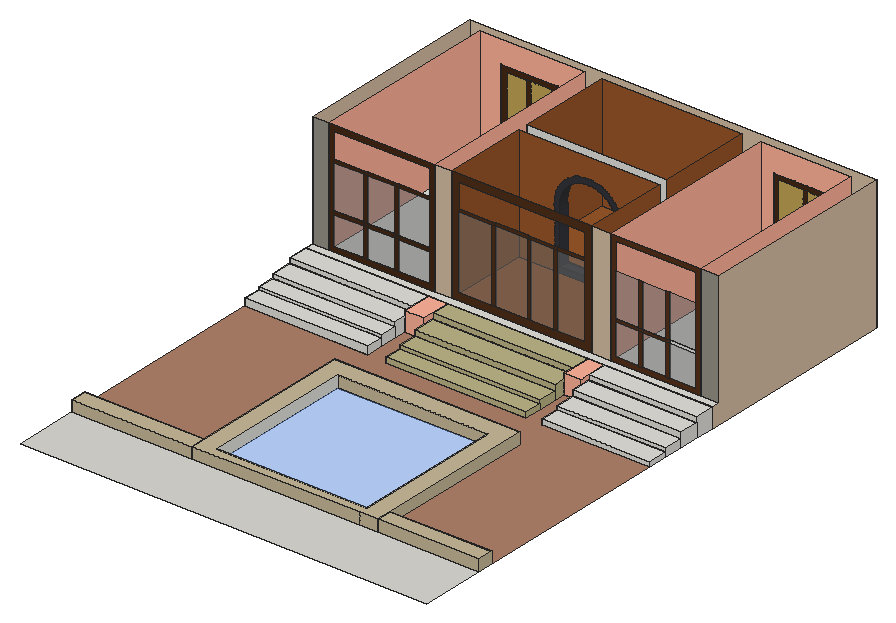
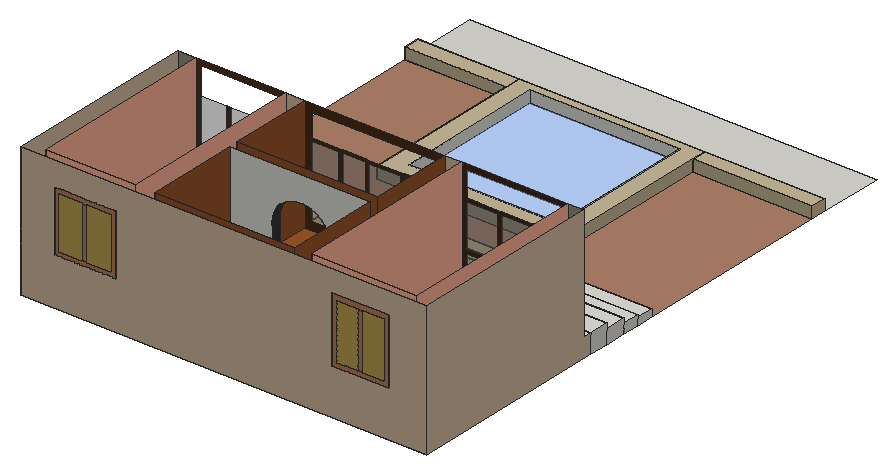
# SketchUp Ruby script. Lengths in inches.
U = 1.inch
M = Sketchup.active_model
def pt(a) = Geom::Point3d.new(a.map { |v| v * U })
def face(e, loops, mat)
  f = e.add_face(loops[0].map { |a| pt(a) })
  loops[1..].each { |l| e.add_face(l.map { |a| pt(a) }).erase! }
  f.material = f.back_material = mat if mat
  f
end
# faces: each face lists its corners as indices into pts; further lists are holes
def faces(e, pts, list, mat = nil) = list.each { |f| face(e, (f[0].is_a?(Array) ? f : [f]).map { |l| l.map { |i| pts[i] } }, mat) }
# xy, xz, yz: faces in a plane at the given z, y or x. An outline is a flat list of corners, or four numbers for a rectangle; further outlines are holes
def ring(l) = l.size == 4 ? [[l[0], l[1]], [l[2], l[1]], [l[2], l[3]], [l[0], l[3]]] : l.each_slice(2).to_a
def flat(e, list, mat, &to3) = list.each { |f| face(e, (f[0].is_a?(Array) ? f : [f]).map { |l| ring(l).map { |u, v| to3.(u, v) } }, mat) }
def xy(e, z, list, mat = nil) = flat(e, list, mat) { |x, y| [x, y, z] }
def xz(e, y, list, mat = nil) = flat(e, list, mat) { |x, z| [x, y, z] }
def yz(e, x, list, mat = nil) = flat(e, list, mat) { |y, z| [x, y, z] }
def lines(e, pts, list) = list.each { |a, b| e.add_line(pt(pts[a]), pt(pts[b])) }
# prism: a flat outline (further loops are holes) pulled along v
def prism(e, loops, v, mat = nil)
  f = face(e, loops, mat); d = Geom::Vector3d.new(v.map { |x| x * U })
  f.pushpull(f.normal.samedirection?(d) ? d.length : -d.length)
end
def box(e, o, s, mat = nil) = prism(e, [[o, [o[0] + s[0], o[1], o[2]], [o[0] + s[0], o[1] + s[1], o[2]], [o[0], o[1] + s[1], o[2]]]], [0, 0, s[2]], mat)
def at(x, y, z, deg = 0) = Geom::Transformation.translation(pt([x, y, z])) * Geom::Transformation.rotation(ORIGIN, Z_AXIS, deg.degrees)
def axes(o, x, y, z) = Geom::Transformation.new([*x, 0, *y, 0, *z, 0, *pt(o).to_a, 1])
def part(name) = M.definitions.add(name)
# library, detail: a bought-in or finely detailed component or shape, given as its bounding box
def library(name, o, s) = part(name).tap { |d| box(d.entities, o, s) }
def detail(e, o, s) = box(e.add_group.entities, o, s)
def put(e, d, t, mat = nil) = e.add_instance(d, t).tap { |i| i.material = mat if mat }
def group(e, t, mat = nil) = e.add_group.tap { |g| g.transformation = t; g.material = mat if mat }.entities
root = M.entities
M.materials.add("[Blinds Cloth Horizontal]").color = [192, 163, 85]
M.materials.add("[Color B02]").color = [255, 178, 153]
M.materials.add("[Formica Beige]").color = [211, 187, 149]
M.materials.add("[Formica Graystone]").color = [149, 146, 135]
M.materials.add("[Formica Laminate Dark]").color = [50, 53, 60]
M.materials.add("[Formica Laminate Light]").color = [213, 189, 164]
M.materials.add("[Marble Carrara Gold Floor Tile]").color = [225, 223, 217]
M.materials.add("[Pavers Driveway Brick]").color = [176, 130, 106]
M.materials.add("[Quartz Light Brown]").color = [199, 184, 152]
M.materials.add("[Terrazzo Tile Light]").color = [219, 217, 210]
M.materials.add("[Tile Ceramic Natural]").color = [189, 180, 134]
M.materials.add("[Translucent Glass Blue]").color = [100, 149, 237]
M.materials["[Translucent Glass Blue]"].alpha = 0.5
M.materials.add("[Translucent Glass Gray]").color = [128, 128, 128]
M.materials["[Translucent Glass Gray]"].alpha = 0.5
M.materials.add("[Wood Cherry Original]").color = [152, 86, 42]
M.materials.add("[Wood Veneer 01]").color = [71, 41, 22]
M.materials.add("[Wood Veneer 01]1").color = [84, 49, 25]
M.materials.add("[Wood Veneer 01]4").color = [79, 46, 24]
M.materials.add("[Wood Veneer 02]").color = [190, 128, 91]
xy(root,-11.1875,[[0,68.19,126.18,84.67],[[126.18,68.19,322.06,256.19],[144.85,77.55,303.39,237.52]],[322.06,68.19,428.94,84.67],[314.84,293.92,428.94,314.25],[150.11,294.5,297.86,312.54],
  [0,296.1,129.48,314.24],[150.11,312.54,297.86,332.92],[0,314.24,129.48,332.39],[314.84,314.25,428.94,334.58],[0,332.39,129.48,354.8],
  [150.11,332.92,297.86,355.84],[314.84,334.58,428.94,355.16],[129.48,344.68,150.11,376.12],[297.86,344.68,314.84,376.12],[0,354.8,129.48,376.12],
  [314.84,355.16,428.94,376.12],[150.11,355.84,297.86,376.12],[0,376.12,428.94,592.14]])
xy(root,-11.1875,[[0,84.67,0,296.1,129.48,296.1,129.48,344.68,150.11,344.68,150.11,294.5,297.86,294.5,297.86,344.68,314.84,344.68,314.84,293.92,428.94,293.92,428.94,84.67,322.06,84.67,322.06,256.19,126.18,256.19,126.18,84.67]],"[Pavers Driveway Brick]")
xy(root,-11.1875,[[0,0,428.94,68.19]],"[Terrazzo Tile Light]")
xy(root,-11.1875,[[144.85,77.55,303.39,237.52]],"[Translucent Glass Blue]")
xy(root,-6.0625,[[314.84,293.92,428.94,314.25]],"[Marble Carrara Gold Floor Tile]")
xy(root,-5.6875,[[150.11,294.5,297.86,312.54]],"[Tile Ceramic Natural]")
xy(root,-3.3125,[[0,296.1,129.48,314.24]],"[Marble Carrara Gold Floor Tile]")
xy(root,-2.5625,[[150.11,312.54,297.86,332.92]],"[Tile Ceramic Natural]")
xy(root,-2.3125,[[314.84,314.25,428.94,334.58]],"[Marble Carrara Gold Floor Tile]")
xy(root,-0.625,[[0,314.24,129.48,332.39]],"[Marble Carrara Gold Floor Tile]")
xy(root,0.8125,[[0,68.19,126.18,84.67],[[126.18,68.19,322.06,256.19],[144.85,77.55,303.39,237.52]],[322.06,68.19,428.94,84.67]],"[Quartz Light Brown]")
xy(root,3.25,[[150.11,332.92,297.86,355.84]],"[Tile Ceramic Natural]")
xy(root,3.625,[[0,332.39,129.48,354.8],[314.84,334.58,428.94,355.16]],"[Marble Carrara Gold Floor Tile]")
xy(root,9,[[17.625,385.12,128.66,583.14],[314.84,385.12,409.38,583.14]])
xy(root,9,[[129.48,344.68,150.11,376.12],[297.86,344.68,314.84,376.12]],"[Color B02]")
xy(root,9,[[0,354.8,129.48,376.12],[314.84,355.16,428.94,376.12],[0,376.12,428.94,385.12]],"[Marble Carrara Gold Floor Tile]")
xy(root,9,[[150.11,355.84,297.86,376.12]],"[Tile Ceramic Natural]")
xy(root,9,[[146.72,385.12,294.66,474.18],[146.72,484.13,294.66,583.14]],"[Wood Cherry Original]")
xy(root,14.86,[[189.8125,474.18,249.22,484.13]],"[Formica Laminate Dark]")
xy(root,37.28,[[40.61,583.14,100.11,592.14]])
xy(root,39.23,[[328.4,583.14,393.03,592.14]])
xz(root,68.19,[[0,-11.1875,126.18,0.8125],[126.18,-11.1875,303.39,0.8125],[303.39,-11.1875,322.06,0.8125],[322.06,-11.1875,428.94,0.8125]],"[Quartz Light Brown]")
xz(root,77.55,[[144.85,-11.1875,303.39,0.8125]])
xz(root,84.67,[[0,-11.1875,126.18,0.8125],[322.06,-11.1875,428.94,0.8125]],"[Quartz Light Brown]")
xz(root,237.52,[[144.85,-11.1875,303.39,0.8125]],"[Quartz Light Brown]")
xz(root,256.19,[[126.18,-11.1875,322.06,0.8125]],"[Quartz Light Brown]")
xz(root,293.92,[[314.84,-11.1875,428.94,-6.0625]],"[Marble Carrara Gold Floor Tile]")
xz(root,294.5,[[150.11,-11.1875,297.86,-5.6875]],"[Tile Ceramic Natural]")
xz(root,296.1,[[0,-11.1875,129.48,-3.3125]],"[Marble Carrara Gold Floor Tile]")
xz(root,312.54,[[150.11,-11.1875,297.86,-5.6875]])
xz(root,312.54,[[150.11,-5.6875,297.86,-2.5625]],"[Tile Ceramic Natural]")
xz(root,314.24,[[0,-11.1875,129.48,-3.3125]])
xz(root,314.24,[[0,-3.3125,129.48,-0.625]],"[Marble Carrara Gold Floor Tile]")
xz(root,314.25,[[314.84,-11.1875,428.94,-6.0625]])
xz(root,314.25,[[314.84,-6.0625,428.94,-2.3125]],"[Marble Carrara Gold Floor Tile]")
xz(root,332.39,[[0,-11.1875,129.48,-0.625]])
xz(root,332.39,[[0,-0.625,129.48,3.625]],"[Marble Carrara Gold Floor Tile]")
xz(root,332.92,[[150.11,-11.1875,297.86,-2.5625]])
xz(root,332.92,[[150.11,-2.5625,297.86,3.25]],"[Tile Ceramic Natural]")
xz(root,334.58,[[314.84,-11.1875,428.94,-2.3125]])
xz(root,334.58,[[314.84,-2.3125,428.94,3.625]],"[Marble Carrara Gold Floor Tile]")
xz(root,344.68,[[129.48,-11.1875,150.11,9],[297.86,-11.1875,314.84,9]],"[Color B02]")
xz(root,354.8,[[0,-11.1875,129.48,3.625]])
xz(root,354.8,[[0,3.625,129.48,9]],"[Marble Carrara Gold Floor Tile]")
xz(root,355.16,[[314.84,-11.1875,428.94,3.625]])
xz(root,355.16,[[314.84,3.625,428.94,9]],"[Marble Carrara Gold Floor Tile]")
xz(root,355.84,[[150.11,-11.1875,297.86,3.25]])
xz(root,355.84,[[150.11,3.25,297.86,9]],"[Tile Ceramic Natural]")
xz(root,376.12,[[0,-11.1875,129.48,9],[129.48,-11.1875,150.11,9],[150.11,-11.1875,297.86,9],[297.86,-11.1875,314.84,9],[314.84,-11.1875,428.94,9]])
xz(root,385.12,[[376.51,47.26,404.48,50.05]])
xz(root,385.12,[[0,9,17.625,129],[409.38,9,428.94,129]],"[Formica Graystone]")
xz(root,385.12,[[128.66,9,146.72,129],[294.66,9,314.84,129]],"[Formica Laminate Light]")
xz(root,385.12,[[319.73,13.89,344.24,47.26],[348.55,13.89,372.21,47.26],[376.51,13.89,404.48,47.26],[22.98,14.36,53.7,44.51],[57.87,14.36,86.41,44.51],
  [90.59,14.36,123.3,44.51],[154.41,16.69,189.27,93.33],[193.22,16.69,226.58,93.33],[230.53,16.69,254.8,93.33],[258.75,16.69,286.96,93.33],
  [22.98,48.14,53.7,93.75],[57.87,48.14,86.41,93.75],[90.59,48.14,123.3,93.75],[319.73,50.05,344.24,95.2],[348.55,50.05,372.21,95.2],
  [376.51,50.05,404.48,95.2]],"[Translucent Glass Gray]")
xz(root,385.12,[[[17.625,9,128.66,129],[22.98,14.36,123.3,123.64]],[53.7,14.36,57.87,44.51],[86.41,14.36,90.59,44.51],[22.98,44.51,53.7,48.14],[53.7,44.51,57.87,48.14],
  [57.87,44.51,86.41,48.14],[86.41,44.51,90.59,48.14],[90.59,44.51,123.3,48.14],[53.7,48.14,57.87,93.75],[86.41,48.14,90.59,93.75],
  [22.98,93.75,53.7,96.89],[53.7,93.75,57.87,96.89],[57.87,93.75,86.41,96.89],[86.41,93.75,90.59,96.89],[90.59,93.75,123.3,96.89]],"[Wood Veneer 01]")
xz(root,385.12,[[[314.84,9,409.38,129],[319.73,13.89,404.48,124.11]],[344.24,13.89,348.55,47.26],[372.21,13.89,376.51,47.26],[319.73,47.26,344.24,50.05],[344.24,47.26,348.55,50.05],
  [348.55,47.26,372.21,50.05],[372.21,47.26,376.51,50.05],[344.24,50.05,348.55,95.2],[372.21,50.05,376.51,95.2]],"[Wood Veneer 01]1")
xz(root,385.12,[[[146.72,9,294.66,129],[154.41,16.69,286.96,121.31]],[189.27,16.69,193.22,93.33],[226.58,16.69,230.53,93.33],[254.8,16.69,258.75,93.33],[154.41,93.33,189.27,96.38],
  [189.27,93.33,193.22,96.38],[193.22,93.33,226.58,96.38],[226.58,93.33,230.53,96.38],[230.53,93.33,254.8,96.38],[254.8,93.33,258.75,96.38],
  [258.75,93.33,286.96,96.38]],"[Wood Veneer 01]4")
xz(root,474.18,[[[183.96,9,255.08,9,255.08,66.625,255.36,68.6875,255.51,70.76,255.55,72.84,255.46,74.92,255.26,76.99,254.93,79.04,254.49,81.08,253.93,83.08,253.26,85.05,252.47,86.97,251.58,88.85,250.58,90.67,249.47,92.43,248.27,94.13,246.97,95.75,245.57,97.3,244.09,98.76,242.53,100.13,240.89,101.42,239.18,102.6,237.41,103.68,235.58,104.67,233.6875,105.54,231.75,106.3,229.78,106.95,227.77,107.48,225.73,107.9,223.67,108.2,221.6,108.38,219.52,108.44,217.44,108.38,215.37,108.2,213.31,107.9,211.27,107.48,209.26,106.95,207.29,106.3,205.35,105.54,203.46,104.67,201.63,103.68,199.85,102.6,198.14,101.42,196.51,100.13,194.94,98.76,193.47,97.3,192.07,95.75,190.77,94.13,189.57,92.43,188.46,90.67,187.46,88.85,186.5625,86.97,185.78,85.05,185.1,83.08,184.55,81.08,184.1,79.04,183.78,76.99,183.58,74.92,183.49,72.84,183.53,70.76,183.68,68.6875,183.96,66.625],[189.8125,14.86,189.8125,67.01,189.51,69.29,189.38,71.03,189.35,72.77,189.42,74.51,189.59,76.24,189.86,77.96,190.23,79.67,190.7,81.34,191.27,82.99,191.92,84.6,192.67,86.18,193.51,87.7,194.4375,89.18,195.45,90.6,196.54,91.96,197.7,93.25,198.94,94.47,200.25,95.625,201.62,96.7,203.05,97.69,204.54,98.6,206.07,99.42,207.66,100.15,209.28,100.79,210.93,101.33,212.61,101.78,214.32,102.13,216.04,102.38,217.78,102.53,219.52,102.58,221.26,102.53,223,102.38,224.72,102.13,226.42,101.78,228.11,101.33,229.76,100.79,231.38,100.15,232.96,99.42,234.5,98.6,235.99,97.69,237.42,96.7,238.79,95.625,240.1,94.47,241.34,93.25,242.5,91.96,243.59,90.6,244.6,89.18,245.53,87.7,246.37,86.18,247.11,84.6,247.77,82.99,248.34,81.34,248.8,79.67,249.17,77.96,249.44,76.24,249.62,74.51,249.6875,72.77,249.66,71.03,249.53,69.29,249.22,67.01,249.22,14.86]]],"[Formica Laminate Dark]")
xz(root,474.18,[[146.72,9,183.96,9,183.96,66.625,183.68,68.6875,183.53,70.76,183.49,72.84,183.58,74.92,183.78,76.99,184.1,79.04,184.55,81.08,185.1,83.08,185.78,85.05,186.5625,86.97,187.46,88.85,188.46,90.67,189.57,92.43,190.77,94.13,192.07,95.75,193.47,97.3,194.94,98.76,196.51,100.13,198.14,101.42,199.85,102.6,201.63,103.68,203.46,104.67,205.35,105.54,207.29,106.3,209.26,106.95,211.27,107.48,213.31,107.9,215.37,108.2,217.44,108.38,219.52,108.44,221.6,108.38,223.67,108.2,225.73,107.9,227.77,107.48,229.78,106.95,231.75,106.3,233.6875,105.54,235.58,104.67,237.41,103.68,239.18,102.6,240.89,101.42,242.53,100.13,244.09,98.76,245.57,97.3,246.97,95.75,248.27,94.13,249.47,92.43,250.58,90.67,251.58,88.85,252.47,86.97,253.26,85.05,253.93,83.08,254.49,81.08,254.93,79.04,255.26,76.99,255.46,74.92,255.55,72.84,255.51,70.76,255.36,68.6875,255.08,66.625,255.08,9,294.66,9,294.66,129,146.72,129]],"[Wood Cherry Original]")
xz(root,484.13,[[[146.72,9,294.66,129],[189.8125,14.86,249.22,14.86,249.22,67.01,249.53,69.29,249.66,71.03,249.6875,72.77,249.62,74.51,249.44,76.24,249.17,77.96,248.8,79.67,248.34,81.34,247.77,82.99,247.11,84.6,246.37,86.18,245.53,87.7,244.6,89.18,243.59,90.6,242.5,91.96,241.34,93.25,240.1,94.47,238.79,95.625,237.42,96.7,235.99,97.69,234.5,98.6,232.96,99.42,231.38,100.15,229.76,100.79,228.11,101.33,226.42,101.78,224.72,102.13,223,102.38,221.26,102.53,219.52,102.58,217.78,102.53,216.04,102.38,214.32,102.13,212.61,101.78,210.93,101.33,209.28,100.79,207.66,100.15,206.07,99.42,204.54,98.6,203.05,97.69,201.62,96.7,200.25,95.625,198.94,94.47,197.7,93.25,196.54,91.96,195.45,90.6,194.4375,89.18,193.51,87.7,192.67,86.18,191.92,84.6,191.27,82.99,190.7,81.34,190.23,79.67,189.86,77.96,189.59,76.24,189.42,74.51,189.35,72.77,189.38,71.03,189.51,69.29,189.8125,67.01]]])
xz(root,583.14,[[46.41,43.08,67.5,100.66],[71.375,43.08,94.31,100.66],[333.21,44.04,358.33,99.04],[363.37,44.04,388.22,99.04]],"[Blinds Cloth Horizontal]")
xz(root,583.14,[[[17.625,9,128.66,129],[40.61,37.28,100.11,106.46]],[[314.84,9,409.38,129],[328.4,39.23,393.03,103.85]]],"[Color B02]")
xz(root,583.14,[[146.72,9,294.66,129]],"[Wood Cherry Original]")
xz(root,583.14,[[[40.61,37.28,100.11,106.46],[46.41,43.08,94.31,100.66]],[[328.4,39.23,393.03,103.85],[333.21,44.04,388.22,99.04]],[67.5,43.08,71.375,100.66],[358.33,44.04,363.37,99.04]],"[Wood Veneer 01]")
xz(root,592.14,[[45.9,42.57,67.42,101.17],[73.22,42.57,94.8125,101.17],[333.59,44.41,358.46,98.67],[364.01,44.41,387.84,98.67]],"[Blinds Cloth Horizontal]")
xz(root,592.14,[[[0,-11.1875,428.94,129],[328.4,39.23,393.03,103.85],[40.61,37.28,100.11,106.46]]],"[Formica Laminate Light]")
xz(root,592.14,[[[40.61,37.28,100.11,106.46],[45.9,42.57,94.8125,101.17]],[[328.4,39.23,393.03,103.85],[333.59,44.41,387.84,98.67]],[67.42,42.57,73.22,101.17],[358.46,44.41,364.01,98.67]],"[Wood Veneer 02]")
yz(root,0,[[68.19,-11.1875,84.67,0.8125]],"[Formica Beige]")
yz(root,0,[[376.12,-11.1875,376.12,9,385.12,9,385.12,129,592.14,129,592.14,-11.1875]],"[Formica Laminate Light]")
yz(root,0,[[296.1,-11.1875,314.24,-3.3125],[314.24,-11.1875,332.39,-0.625],[332.39,-11.1875,354.8,3.625],[354.8,-11.1875,376.12,9]],"[Marble Carrara Gold Floor Tile]")
yz(root,17.625,[[385.12,9,583.14,129]],"[Color B02]")
yz(root,40.61,[[583.14,37.28,592.14,106.46]])
yz(root,100.11,[[583.14,37.28,592.14,106.46]])
yz(root,126.18,[[68.19,-11.1875,84.67,0.8125]])
yz(root,126.18,[[84.67,-11.1875,256.19,0.8125]],"[Quartz Light Brown]")
yz(root,128.66,[[385.12,9,583.14,129]],"[Color B02]")
yz(root,129.48,[[344.68,-11.1875,354.8,3.625],[354.8,-11.1875,376.12,9]])
yz(root,129.48,[[344.68,3.625,354.8,9]],"[Color B02]")
yz(root,129.48,[[296.1,-11.1875,314.24,-3.3125],[314.24,-11.1875,332.39,-0.625],[332.39,-11.1875,344.68,3.625]],"[Marble Carrara Gold Floor Tile]")
yz(root,144.85,[[77.55,-11.1875,237.52,0.8125]])
yz(root,146.72,[[385.12,9,474.18,129],[484.13,9,583.14,129]],"[Wood Cherry Original]")
yz(root,150.11,[[344.68,-11.1875,355.84,3.25],[355.84,-11.1875,376.12,9]])
yz(root,150.11,[[344.68,3.25,355.84,9]],"[Color B02]")
yz(root,150.11,[[294.5,-11.1875,312.54,-5.6875],[312.54,-11.1875,332.92,-2.5625],[332.92,-11.1875,344.68,3.25]],"[Tile Ceramic Natural]")
yz(root,189.8125,[[474.18,14.86,484.13,67.01]],"[Formica Laminate Dark]")
yz(root,249.22,[[474.18,14.86,484.13,67.01]],"[Formica Laminate Dark]")
yz(root,294.66,[[385.12,9,474.18,129],[484.13,9,583.14,129]],"[Wood Cherry Original]")
yz(root,297.86,[[344.68,-11.1875,355.84,3.25],[355.84,-11.1875,376.12,9]])
yz(root,297.86,[[344.68,3.25,355.84,9]],"[Color B02]")
yz(root,297.86,[[294.5,-11.1875,312.54,-5.6875],[312.54,-11.1875,332.92,-2.5625],[332.92,-11.1875,344.68,3.25]],"[Tile Ceramic Natural]")
yz(root,303.39,[[77.55,-11.1875,237.52,0.8125]])
yz(root,314.84,[[344.68,-11.1875,355.16,3.625],[355.16,-11.1875,376.12,9]])
yz(root,314.84,[[344.68,3.625,355.16,9],[385.12,9,583.14,129]],"[Color B02]")
yz(root,314.84,[[293.92,-11.1875,314.25,-6.0625],[314.25,-11.1875,334.58,-2.3125],[334.58,-11.1875,344.68,3.625]],"[Marble Carrara Gold Floor Tile]")
yz(root,322.06,[[68.19,-11.1875,84.67,0.8125]])
yz(root,322.06,[[84.67,-11.1875,256.19,0.8125]],"[Quartz Light Brown]")
yz(root,328.4,[[583.14,39.23,592.14,103.85]])
yz(root,393.03,[[583.14,39.23,592.14,103.85]])
yz(root,409.38,[[385.12,9,583.14,129]],"[Color B02]")
yz(root,428.94,[[376.12,-11.1875,592.14,-11.1875,592.14,129,385.12,129,385.12,9,376.12,9]],"[Formica Laminate Light]")
yz(root,428.94,[[293.92,-11.1875,314.25,-6.0625],[314.25,-11.1875,334.58,-2.3125],[334.58,-11.1875,355.16,3.625],[355.16,-11.1875,376.12,9]],"[Marble Carrara Gold Floor Tile]")
yz(root,428.94,[[68.19,-11.1875,84.67,0.8125]],"[Quartz Light Brown]")
p = [[189.51,474.18,69.29],[189.8125,474.18,67.01],[189.8125,484.13,67.01],[189.51,484.13,69.29],[249.22,474.18,67.01],[249.53,474.18,69.29],
  [249.53,484.13,69.29],[249.22,484.13,67.01],[189.38,474.18,71.03],[189.38,484.13,71.03],[249.66,474.18,71.03],[249.66,484.13,71.03],
  [189.35,474.18,72.77],[189.35,484.13,72.77],[249.6875,474.18,72.77],[249.6875,484.13,72.77],[189.42,474.18,74.51],[189.42,484.13,74.51],
  [249.62,474.18,74.51],[249.62,484.13,74.51],[189.59,474.18,76.24],[189.59,484.13,76.24],[249.44,474.18,76.24],[249.44,484.13,76.24],
  [189.86,474.18,77.96],[189.86,484.13,77.96],[249.17,474.18,77.96],[249.17,484.13,77.96],[190.23,474.18,79.67],[190.23,484.13,79.67],
  [248.8,474.18,79.67],[248.8,484.13,79.67],[190.7,474.18,81.34],[190.7,484.13,81.34],[248.34,474.18,81.34],[248.34,484.13,81.34],
  [191.27,474.18,82.99],[191.27,484.13,82.99],[247.77,474.18,82.99],[247.77,484.13,82.99],[191.92,474.18,84.6],[191.92,484.13,84.6],
  [247.11,474.18,84.6],[247.11,484.13,84.6],[192.67,474.18,86.18],[192.67,484.13,86.18],[246.37,474.18,86.18],[246.37,484.13,86.18],
  [193.51,474.18,87.7],[193.51,484.13,87.7],[245.53,474.18,87.7],[245.53,484.13,87.7],[194.4375,474.18,89.18],[194.4375,484.13,89.18],
  [244.6,474.18,89.18],[244.6,484.13,89.18],[195.45,474.18,90.6],[195.45,484.13,90.6],[243.59,474.18,90.6],[243.59,484.13,90.6],
  [196.54,474.18,91.96],[196.54,484.13,91.96],[242.5,474.18,91.96],[242.5,484.13,91.96],[197.7,474.18,93.25],[197.7,484.13,93.25],
  [241.34,474.18,93.25],[241.34,484.13,93.25],[198.94,474.18,94.47],[198.94,484.13,94.47],[240.1,474.18,94.47],[240.1,484.13,94.47]]
faces(root,p,[[0,1,2,3],[4,5,6,7],[8,0,3,9],[5,10,11,6],[12,8,9,13],[10,14,15,11],[16,12,13,17],[14,18,19,15],
  [20,16,17,21],[18,22,23,19],[24,20,21,25],[22,26,27,23],[28,24,25,29],[26,30,31,27],[32,28,29,33],[30,34,35,31],
  [36,32,33,37],[34,38,39,35],[40,36,37,41],[38,42,43,39],[44,40,41,45],[42,46,47,43],[48,44,45,49],[46,50,51,47],
  [52,48,49,53],[50,54,55,51],[56,52,53,57],[54,58,59,55],[60,56,57,61],[58,62,63,59],[64,60,61,65],[62,66,67,63],
  [68,64,65,69],[66,70,71,67]],"[Formica Laminate Dark]")
